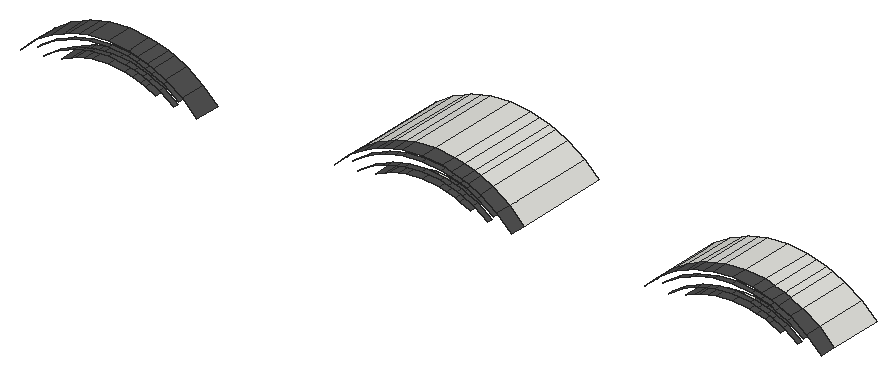
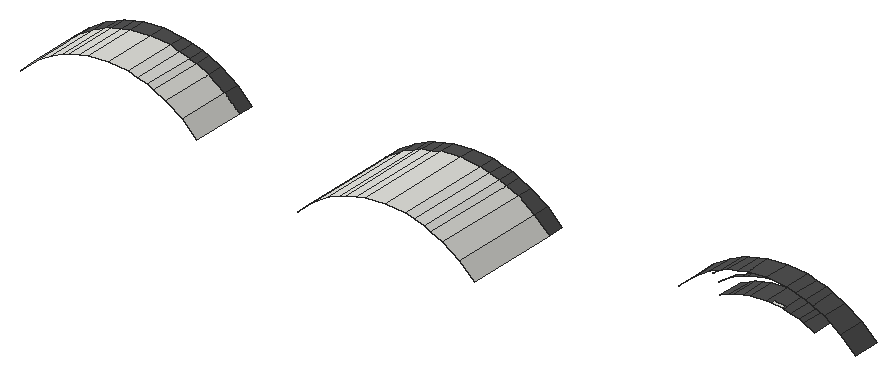
# SketchUp Ruby script. Lengths in inches.
U = 1.inch
M = Sketchup.active_model
def pt(a) = Geom::Point3d.new(a.map { |v| v * U })
def face(e, loops, mat)
  f = e.add_face(loops[0].map { |a| pt(a) })
  loops[1..].each { |l| e.add_face(l.map { |a| pt(a) }).erase! }
  f.material = f.back_material = mat if mat
  f
end
# faces: each face lists its corners as indices into pts; further lists are holes
def faces(e, pts, list, mat = nil) = list.each { |f| face(e, (f[0].is_a?(Array) ? f : [f]).map { |l| l.map { |i| pts[i] } }, mat) }
# xy, xz, yz: faces in a plane at the given z, y or x. An outline is a flat list of corners, or four numbers for a rectangle; further outlines are holes
def ring(l) = l.size == 4 ? [[l[0], l[1]], [l[2], l[1]], [l[2], l[3]], [l[0], l[3]]] : l.each_slice(2).to_a
def flat(e, list, mat, &to3) = list.each { |f| face(e, (f[0].is_a?(Array) ? f : [f]).map { |l| ring(l).map { |u, v| to3.(u, v) } }, mat) }
def xy(e, z, list, mat = nil) = flat(e, list, mat) { |x, y| [x, y, z] }
def xz(e, y, list, mat = nil) = flat(e, list, mat) { |x, z| [x, y, z] }
def yz(e, x, list, mat = nil) = flat(e, list, mat) { |y, z| [x, y, z] }
def lines(e, pts, list) = list.each { |a, b| e.add_line(pt(pts[a]), pt(pts[b])) }
# prism: a flat outline (further loops are holes) pulled along v
def prism(e, loops, v, mat = nil)
  f = face(e, loops, mat); d = Geom::Vector3d.new(v.map { |x| x * U })
  f.pushpull(f.normal.samedirection?(d) ? d.length : -d.length)
end
def box(e, o, s, mat = nil) = prism(e, [[o, [o[0] + s[0], o[1], o[2]], [o[0] + s[0], o[1] + s[1], o[2]], [o[0], o[1] + s[1], o[2]]]], [0, 0, s[2]], mat)
def at(x, y, z, deg = 0) = Geom::Transformation.translation(pt([x, y, z])) * Geom::Transformation.rotation(ORIGIN, Z_AXIS, deg.degrees)
def axes(o, x, y, z) = Geom::Transformation.new([*x, 0, *y, 0, *z, 0, *pt(o).to_a, 1])
def part(name) = M.definitions.add(name)
# library, detail: a bought-in or finely detailed component or shape, given as its bounding box
def library(name, o, s) = part(name).tap { |d| box(d.entities, o, s) }
def detail(e, o, s) = box(e.add_group.entities, o, s)
def put(e, d, t, mat = nil) = e.add_instance(d, t).tap { |i| i.material = mat if mat }
def group(e, t, mat = nil) = e.add_group.tap { |g| g.transformation = t; g.material = mat if mat }.entities
root = M.entities
M.materials.add("[0135_DarkGray]").color = [81, 81, 81]
p = [[82.28,49.6875,744.61],[73.8125,49.6875,736.74],[73.8125,34.6875,736.74],[82.28,34.6875,744.61],[176.65,49.6875,736.74],[168.18,49.6875,744.61],
  [168.18,34.6875,744.61],[176.65,34.6875,736.74],[260.22,49.6875,744.61],[251.75,49.6875,736.74],[251.75,40.6875,736.74],[260.22,40.6875,744.61],
  [354.58,49.6875,736.74],[346.11,49.6875,744.61],[346.11,40.6875,744.61],[354.58,40.6875,736.74],[432,49.6875,736.74],[440.47,49.6875,744.61],
  [440.47,40.6875,744.61],[432,40.6875,736.74],[526.36,49.6875,744.61],[534.83,49.6875,736.74],[534.83,40.6875,736.74],[526.36,40.6875,744.61],
  [251.75,104.375,736.74],[260.22,104.375,744.61],[346.11,104.375,744.61],[354.58,104.375,736.74],[432,80.4375,736.74],[440.47,80.4375,744.61],
  [526.36,80.4375,744.61],[534.83,80.4375,736.74],[454.23,43.6875,743.43],[445.77,43.6875,737.85],[445.77,40.6875,737.85],[454.23,40.6875,743.43],
  [521.06,43.6875,737.85],[512.6,43.6875,743.43],[512.6,40.6875,743.43],[521.06,40.6875,737.85],[273.87,43.6875,743.63],[265.37,43.6875,738.04],
  [265.37,40.6875,738.04],[273.87,40.6875,743.63],[340.96,43.6875,738.04],[332.46,43.6875,743.63],[332.46,40.6875,743.63],[340.96,40.6875,738.04],
  [95.81,37.6875,743.85],[87.28,37.6875,738.24],[87.28,34.6875,738.24],[95.81,34.6875,743.85],[163.18,37.6875,738.24],[154.65,37.6875,743.85],
  [154.65,34.6875,743.85],[163.18,34.6875,738.24],[97.7,49.6875,740.39],[103.75,49.6875,743.0625],[103.75,34.6875,743.0625],[97.7,34.6875,740.39],
  [146.71,49.6875,743.0625],[152.76,49.6875,740.39],[152.76,34.6875,740.39],[146.71,34.6875,743.0625],[275.64,49.6875,740.39],[281.68,49.6875,743.0625],
  [281.68,40.6875,743.0625],[275.64,40.6875,740.39],[324.65,49.6875,743.0625],[330.7,49.6875,740.39],[330.7,40.6875,740.39],[324.65,40.6875,743.0625],
  [455.89,49.6875,740.39],[461.93,49.6875,743.0625],[461.93,40.6875,743.0625],[455.89,40.6875,740.39],[504.9,49.6875,743.0625],[510.95,49.6875,740.39],
  [510.95,40.6875,740.39],[504.9,40.6875,743.0625],[442.54,43.6875,741.96],[451.73,43.6875,748.01],[451.73,40.6875,748.01],[442.54,40.6875,741.96],
  [515.1,43.6875,748.01],[524.29,43.6875,741.96],[524.29,40.6875,741.96],[515.1,40.6875,748.01],[84.26,37.6875,742.08],[93.47,37.6875,748.14],
  [93.47,34.6875,748.14],[84.26,34.6875,742.08],[156.99,37.6875,748.14],[166.19,37.6875,742.08],[166.19,34.6875,742.08],[156.99,34.6875,748.14],
  [262.04,43.6875,742.29],[271.28,43.6875,748.38],[271.28,40.6875,748.38],[262.04,40.6875,742.29],[335.05,43.6875,748.38],[344.3,43.6875,742.29],
  [344.3,40.6875,742.29],[335.05,40.6875,748.38],[106.44,49.6875,744.25],[106.44,34.6875,744.25],[144.02,49.6875,744.25],[144.02,34.6875,744.25],
  [284.38,49.6875,744.25],[284.38,40.6875,744.25],[321.95,49.6875,744.25],[321.95,40.6875,744.25],[464.63,49.6875,744.25],[464.63,40.6875,744.25],
  [502.2,49.6875,744.25],[502.2,40.6875,744.25],[460.54,43.6875,746.21],[460.54,40.6875,746.21],[506.29,43.6875,746.21],[506.29,40.6875,746.21],
  [280.2,43.6875,746.43],[280.2,40.6875,746.43],[326.14,43.6875,746.43],[326.14,40.6875,746.43],[102.16,37.6875,746.66],[102.16,34.6875,746.66],
  [148.3,37.6875,746.66],[148.3,34.6875,746.66],[111.33,49.6875,745.5],[111.33,34.6875,745.5],[139.12,49.6875,745.5],[139.12,34.6875,745.5],
  [289.27,49.6875,745.5],[289.27,40.6875,745.5],[317.06,49.6875,745.5],[317.06,40.6875,745.5],[469.52,49.6875,745.5],[469.52,40.6875,745.5],
  [497.31,49.6875,745.5],[497.31,40.6875,745.5],[91.93,49.6875,750.96],[91.93,34.6875,750.96],[158.52,49.6875,750.96],[158.52,34.6875,750.96],
  [269.87,49.6875,750.96],[269.87,40.6875,750.96],[336.46,49.6875,750.96],[336.46,40.6875,750.96],[450.12,49.6875,750.96],[450.12,40.6875,750.96],
  [516.71,49.6875,750.96],[516.71,40.6875,750.96],[269.87,104.375,750.96],[336.46,104.375,750.96],[450.12,80.4375,750.96],[516.71,80.4375,750.96],
  [115.7,49.6875,746.61],[115.7,34.6875,746.61],[134.75,49.6875,746.61],[134.75,34.6875,746.61],[293.64,49.6875,746.61],[293.64,40.6875,746.61],
  [312.69,49.6875,746.61],[312.69,40.6875,746.61],[473.89,49.6875,746.61],[473.89,40.6875,746.61],[492.94,49.6875,746.61],[492.94,40.6875,746.61],
  [463.5,43.6875,747.52],[463.5,40.6875,747.52],[503.33,43.6875,747.52],[503.33,40.6875,747.52],[283.17,43.6875,747.74],[283.17,40.6875,747.74],
  [323.16,43.6875,747.74],[323.16,40.6875,747.74],[116.29,49.6875,746.66],[116.29,47.6875,746.66],[122.29,47.6875,747.16],[122.29,49.6875,747.16],
  [125.23,49.6875,747.41],[125.23,34.6875,747.41],[303.17,49.6875,747.41],[303.17,40.6875,747.41],[305.64,49.6875,747.2],[305.64,47.6875,747.2],
  [311.64,47.6875,746.7],[311.64,49.6875,746.7],[483.42,49.6875,747.41],[483.42,40.6875,747.41],[483.7,49.6875,747.38],[483.7,47.6875,747.38],
  [489.7,47.6875,746.88],[489.7,49.6875,746.88],[105.15,37.6875,747.98],[105.15,34.6875,747.98],[145.3,37.6875,747.98],[145.3,34.6875,747.98],
  [468.67,43.6875,748.84],[468.67,40.6875,748.84],[498.16,43.6875,748.84],[498.16,40.6875,748.84],[288.36,43.6875,749.07],[288.36,40.6875,749.07],
  [317.97,43.6875,749.07],[317.97,40.6875,749.07],[110.36,37.6875,749.31],[110.36,34.6875,749.31],[140.09,37.6875,749.31],[140.09,34.6875,749.31],
  [458.4375,43.6875,750.98],[458.4375,40.6875,750.98],[508.39,43.6875,750.98],[508.39,40.6875,750.98],[100.19,37.6875,751.11],[100.19,34.6875,751.11],
  [150.27,37.6875,751.11],[150.27,34.6875,751.11],[278.02,43.6875,751.35],[278.02,40.6875,751.35],[328.3125,43.6875,751.35],[328.3125,40.6875,751.35],
  [473.32,43.6875,750.02],[473.32,40.6875,750.02],[493.51,43.6875,750.02],[493.51,40.6875,750.02],[293.03,43.6875,750.26],[293.03,40.6875,750.26],
  [313.3,43.6875,750.26],[313.3,40.6875,750.26],[115.05,37.6875,750.5],[115.05,34.6875,750.5],[135.41,37.6875,750.5],[135.41,34.6875,750.5],
  [483.42,43.6875,750.87],[483.42,40.6875,750.87],[303.17,43.6875,751.1],[303.17,40.6875,751.1],[125.23,37.6875,751.35],[125.23,34.6875,751.35],
  [98.9,49.6875,754.04],[98.9,34.6875,754.04],[151.56,49.6875,754.04],[151.56,34.6875,754.04],[276.84,49.6875,754.04],[276.84,40.6875,754.04],
  [329.5,49.6875,754.04],[329.5,40.6875,754.04],[457.09,49.6875,754.04],[457.09,40.6875,754.04],[461.79,43.6875,752.46],[461.79,40.6875,752.46],
  [505.04,43.6875,752.46],[505.04,40.6875,752.46],[509.75,49.6875,754.04],[509.75,40.6875,754.04],[276.84,104.375,754.04],[329.5,104.375,754.04],
  [457.09,80.4375,754.04],[509.75,80.4375,754.04],[103.56,37.6875,752.6],[103.56,34.6875,752.6],[146.9,37.6875,752.6],[146.9,34.6875,752.6],
  [281.41,43.6875,752.85],[281.41,40.6875,752.85],[324.92,43.6875,752.85],[324.92,40.6875,752.85],[467.39,43.6875,753.88],[467.39,40.6875,753.88],
  [499.45,43.6875,753.88],[499.45,40.6875,753.88],[109.16,37.6875,754.03],[109.16,34.6875,754.03],[141.3,37.6875,754.03],[141.3,34.6875,754.03],
  [287.03,43.6875,754.28],[287.03,40.6875,754.28],[319.3,43.6875,754.28],[319.3,40.6875,754.28],[472.45,43.6875,755.17],[472.45,40.6875,755.17],
  [494.38,43.6875,755.17],[494.38,40.6875,755.17],[102.51,49.6875,755.63],[102.51,34.6875,755.63],[114.24,37.6875,755.32],[114.24,34.6875,755.32],
  [136.22,37.6875,755.32],[136.22,34.6875,755.32],[147.95,49.6875,755.63],[147.95,34.6875,755.63],[280.45,49.6875,755.63],[280.45,40.6875,755.63],
  [325.89,49.6875,755.63],[325.89,40.6875,755.63],[460.7,49.6875,755.63],[460.7,40.6875,755.63],[506.14,49.6875,755.63],[506.14,40.6875,755.63],
  [280.45,104.375,755.63],[325.89,104.375,755.63],[460.7,80.4375,755.63],[506.14,80.4375,755.63],[292.13,43.6875,755.58],[292.13,40.6875,755.58],
  [314.2,43.6875,755.58],[314.2,40.6875,755.58],[483.42,43.6875,756.09],[483.42,40.6875,756.09],[125.23,37.6875,756.24],[125.23,34.6875,756.24],
  [108.37,49.6875,757.13],[108.37,34.6875,757.13],[142.09,49.6875,757.13],[142.09,34.6875,757.13],[286.31,49.6875,757.13],[286.31,40.6875,757.13],
  [303.17,43.6875,756.5],[303.17,40.6875,756.5],[320.02,49.6875,757.13],[320.02,40.6875,757.13],[466.56,49.6875,757.13],[466.56,40.6875,757.13],
  [500.27,49.6875,757.13],[500.27,40.6875,757.13],[286.31,104.375,757.13],[320.02,104.375,757.13],[466.56,80.4375,757.13],[500.27,80.4375,757.13],
  [113.71,49.6875,758.49],[113.71,34.6875,758.49],[136.75,49.6875,758.49],[136.75,34.6875,758.49],[291.65,49.6875,758.49],[291.65,40.6875,758.49],
  [314.6875,49.6875,758.49],[314.6875,40.6875,758.49],[471.9,49.6875,758.49],[471.9,40.6875,758.49],[494.9375,49.6875,758.49],[494.9375,40.6875,758.49],
  [291.65,104.375,758.49],[314.6875,104.375,758.49],[471.9,80.4375,758.49],[494.9375,80.4375,758.49],[125.23,49.6875,759.45],[125.23,34.6875,759.45],
  [303.17,49.6875,759.45],[303.17,40.6875,759.45],[483.42,49.6875,759.45],[483.42,40.6875,759.45],[303.17,104.375,759.45],[483.42,80.4375,759.45],
  [311.64,49.6875,747.2]]
faces(root,p,[[0,1,2,3],[4,5,6,7],[8,9,10,11],[12,13,14,15],[16,17,18,19],[20,21,22,23],[32,33,34,35],[36,37,38,39],
  [40,41,42,43],[44,45,46,47],[48,49,50,51],[52,53,54,55],[56,57,58,59],[60,61,62,63],[64,65,66,67],[68,69,70,71],
  [72,73,74,75],[76,77,78,79],[80,81,82,83],[84,85,86,87],[88,89,90,91],[92,93,94,95],[96,97,98,99],[100,101,102,103],
  [57,104,105,58],[106,60,63,107],[65,108,109,66],[110,68,71,111],[73,112,113,74],[114,76,79,115],[116,32,35,117],[37,118,119,38],
  [120,40,43,121],[45,122,123,46],[124,48,51,125],[53,126,127,54],[104,128,129,105],[130,106,107,131],[108,132,133,109],[134,110,111,135],
  [112,136,137,113],[138,114,115,139],[140,0,3,141],[5,142,143,6],[144,8,11,145],[13,146,147,14],[17,148,149,18],[150,20,23,151],
  [128,156,157,129],[158,130,131,159],[132,160,161,133],[162,134,135,163],[136,164,165,137],[166,138,139,167],[168,116,117,169],[118,170,171,119],
  [172,120,121,173],[122,174,175,123],[156,176,177,178,179,180,181,157],[180,158,159,181],[160,182,183,161],[182,184,185,186,187,162,163,183],[164,188,189,165],[188,190,191,192,193,166,167,189],
  [194,124,125,195],[126,196,197,127],[198,168,169,199],[170,200,201,171],[202,172,173,203],[174,204,205,175],[206,194,195,207],[196,208,209,197],
  [81,210,211,82],[212,84,87,213],[89,214,215,90],[216,92,95,217],[97,218,219,98],[220,100,103,221],[222,198,199,223],[200,224,225,201],
  [226,202,203,227],[204,228,229,205],[230,206,207,231],[208,232,233,209],[234,222,223,235],[224,234,235,225],[236,226,227,237],[228,236,237,229],
  [238,230,231,239],[232,238,239,233],[240,140,141,241],[142,242,243,143],[244,144,145,245],[146,246,247,147],[148,248,249,149],[210,250,251,211],
  [252,212,213,253],[254,150,151,255],[214,260,261,215],[262,216,217,263],[218,264,265,219],[266,220,221,267],[250,268,269,251],[270,252,253,271],
  [260,272,273,261],[274,262,263,275],[264,276,277,265],[278,266,267,279],[268,280,281,269],[282,270,271,283],[284,240,241,285],[272,286,287,273],
  [288,274,275,289],[242,290,291,243],[292,244,245,293],[246,294,295,247],[248,296,297,249],[298,254,255,299],[276,304,305,277],[306,278,279,307],
  [280,308,309,281],[308,282,283,309],[286,310,311,287],[310,288,289,311],[312,284,285,313],[290,314,315,291],[316,292,293,317],[304,318,319,305],
  [318,306,307,319],[294,320,321,295],[296,322,323,297],[324,298,299,325],[330,312,313,331],[314,332,333,315],[334,316,317,335],[320,336,337,321],
  [322,338,339,323],[340,324,325,341],[346,330,331,347],[332,346,347,333],[348,334,335,349],[336,348,349,337],[338,350,351,339],[350,340,341,351]],"[0135_DarkGray]")
faces(root,p,[[8,9,24,25],[12,13,26,27],[17,16,28,29],[21,20,30,31],[144,8,25,152],[13,146,153,26],[148,17,29,154],[20,150,155,30],
  [176,179,178,177],[184,187,186,185],[190,193,192,191],[244,144,152,256],[146,246,257,153],[248,148,154,258],[150,254,259,155],[292,244,256,300],
  [246,294,301,257],[296,248,258,302],[254,298,303,259],[316,292,300,326],[294,320,327,301],[322,296,302,328],[298,324,329,303],[334,316,326,342],
  [320,336,343,327],[338,322,328,344],[324,340,345,329],[348,334,342,352],[336,348,352,343],[350,338,344,353],[340,350,353,345]])
lines(root,p,[[187,354]])
